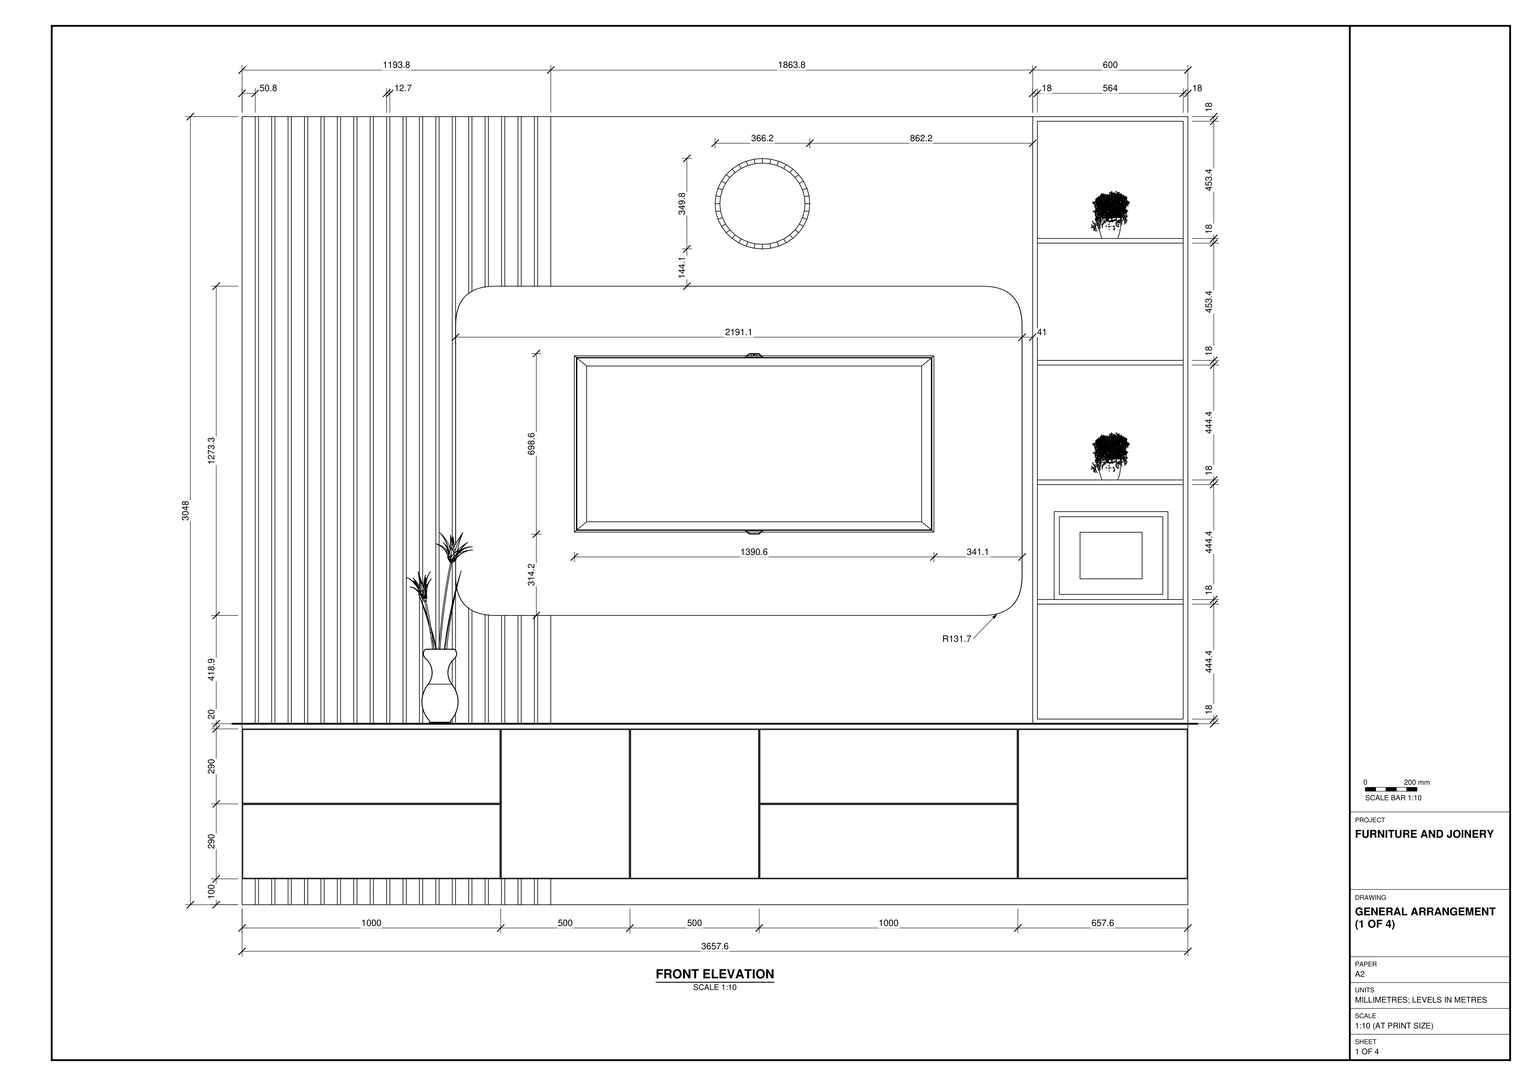
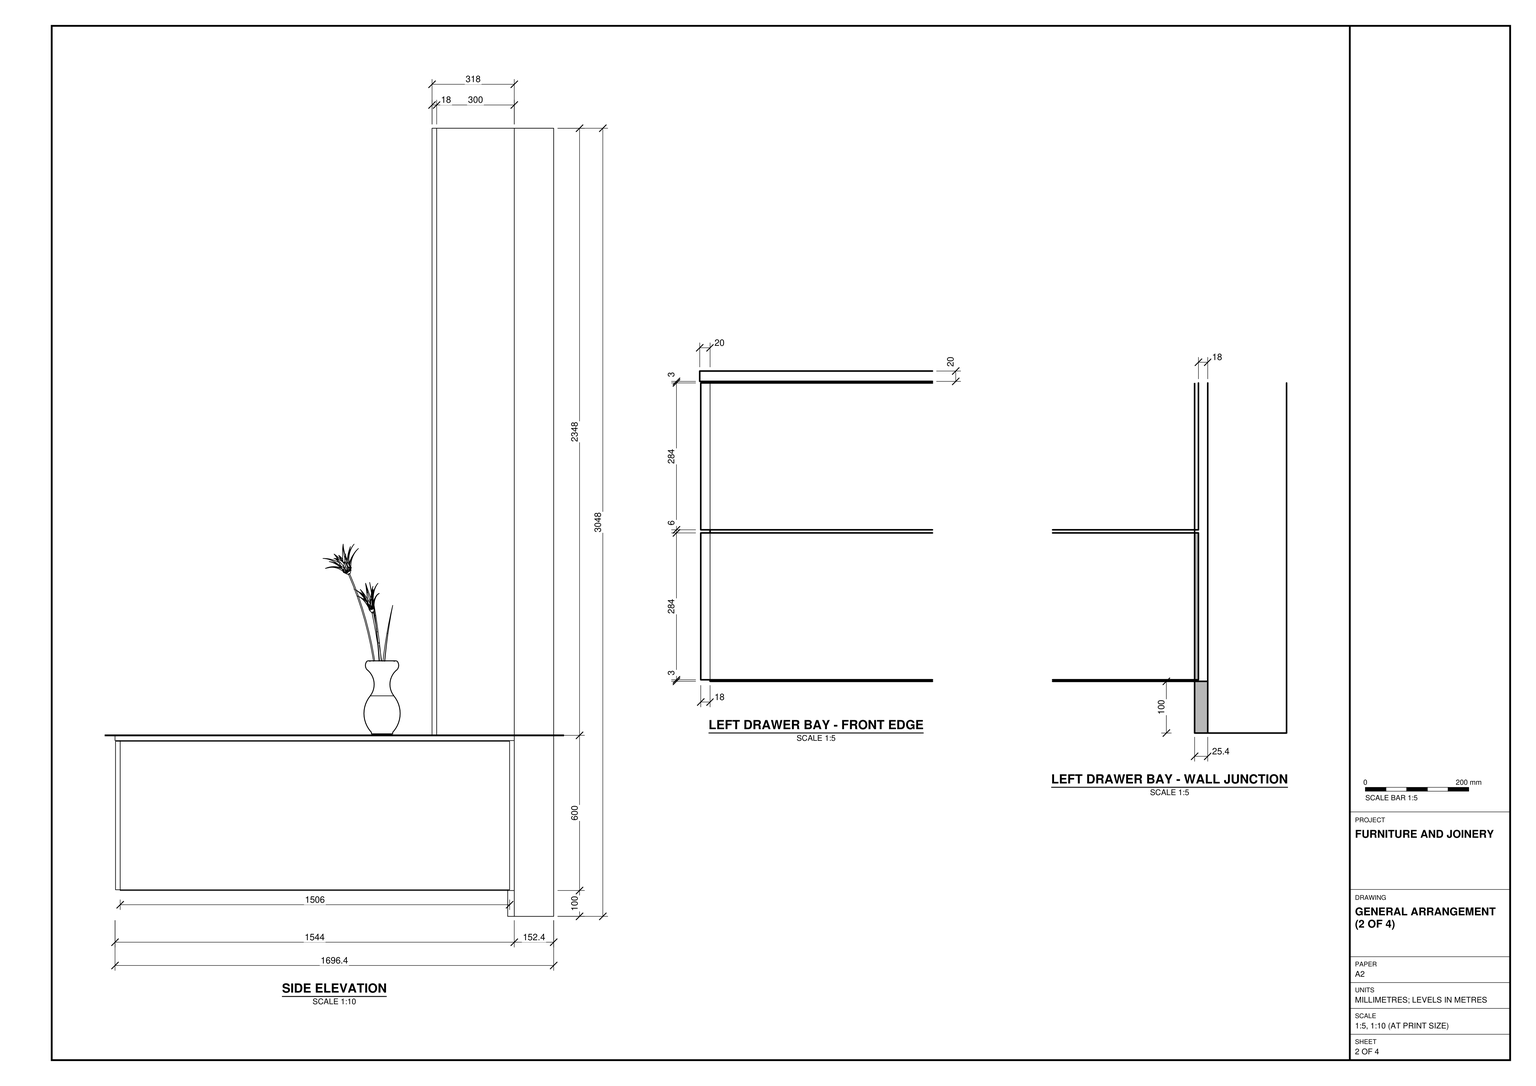
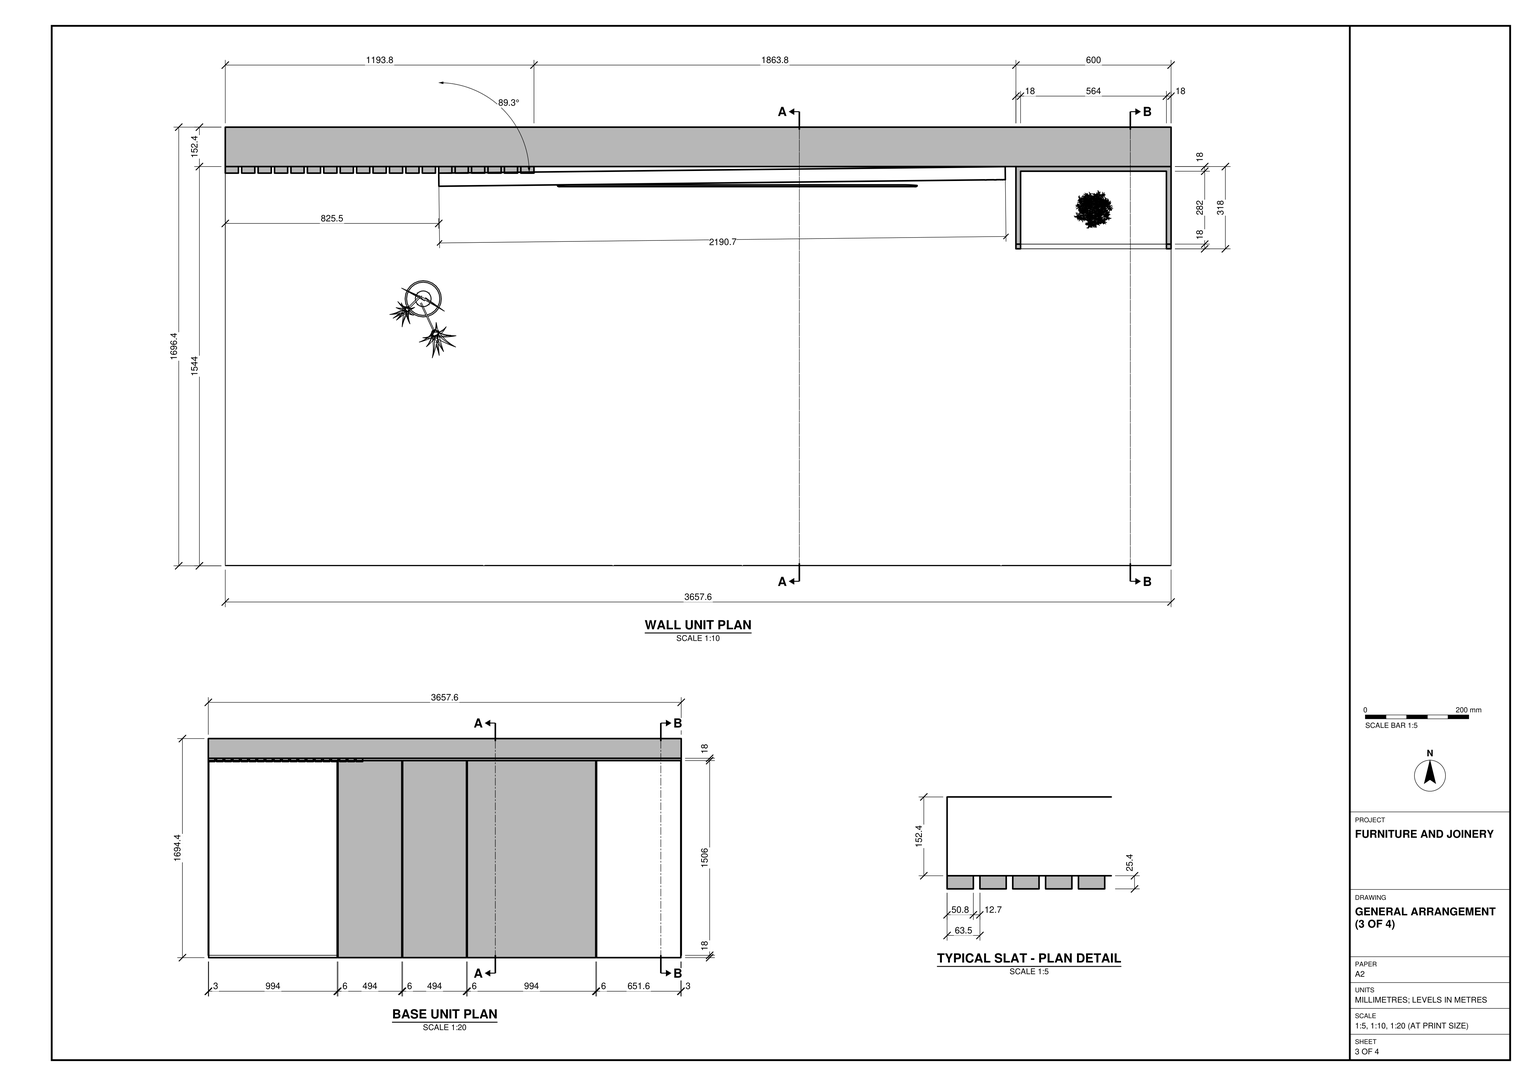
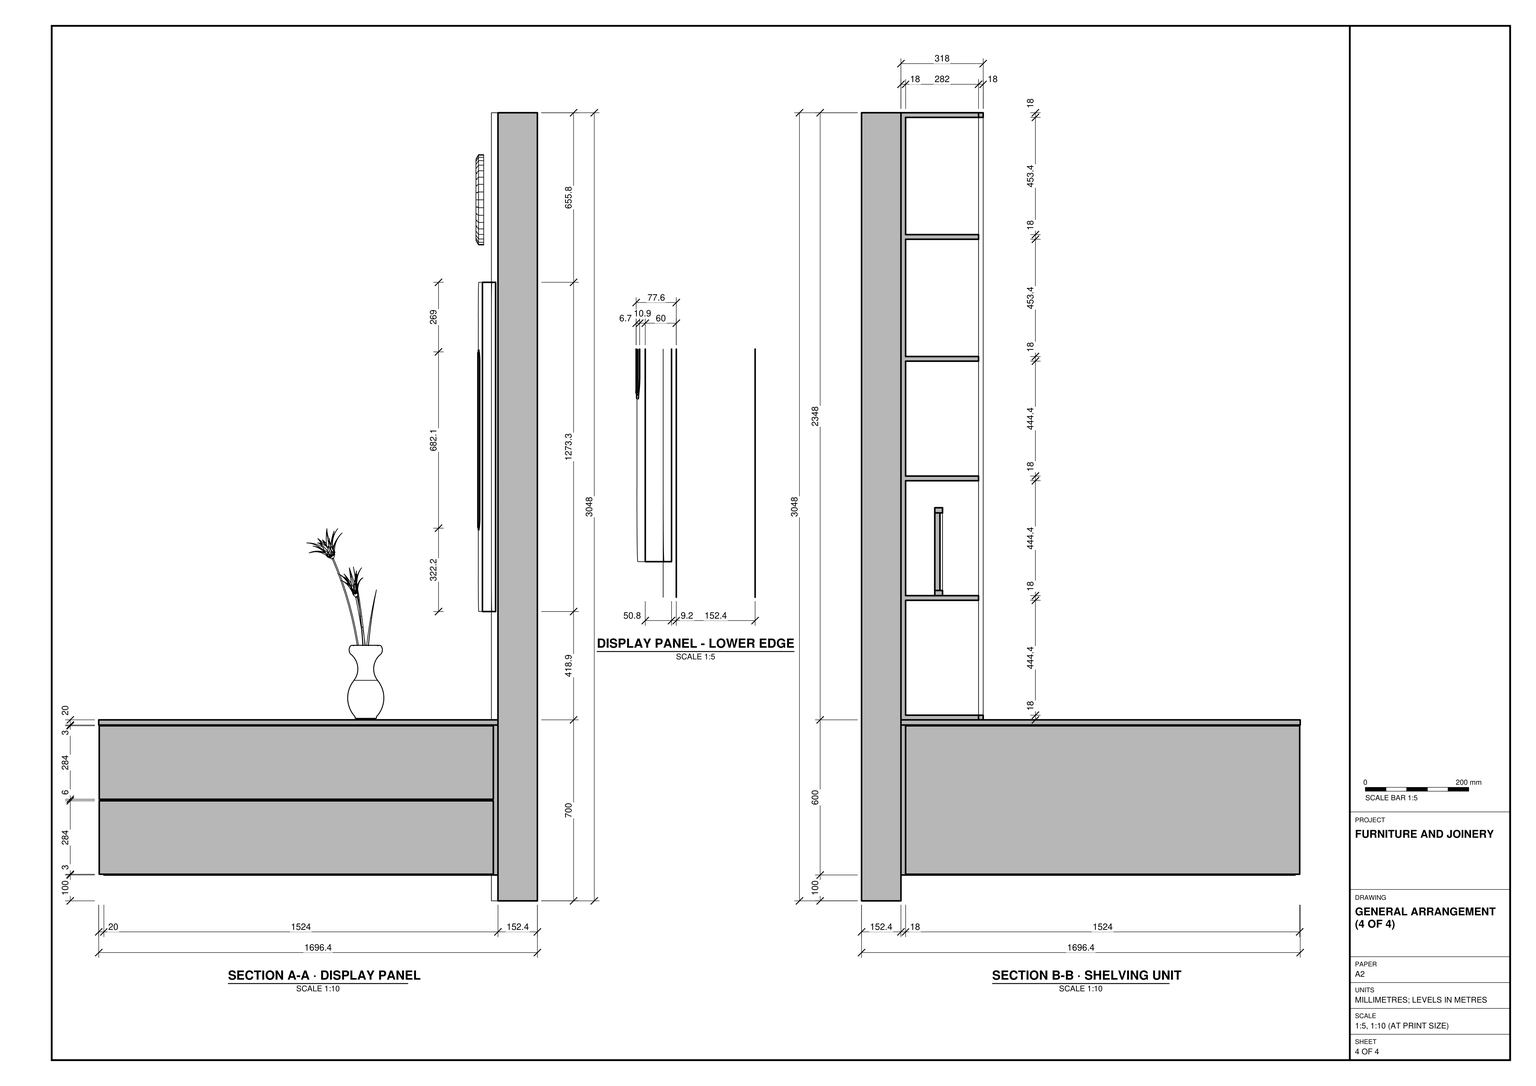
Build the TV wall unit in SketchUp from task_files/diagram_01.pdf. Work in millimetres, using the single floor level at 0 mm as the height datum. The complete assembly is 3657.6 mm wide, 1696.4 mm deep and 3048 mm high. Include the 152.4 mm thick backing wall; the overall depth includes this wall.

Run the base cabinetry across the full width, leaving its underside 100 mm above the floor. Model the continuous 20 mm thick top and follow the front elevation for the bay widths. The two wide bays have stacked drawer fronts, while the narrower bays have full-height fronts. Use the enlarged drawer detail for the gaps around the fronts.

On the left, model the vertical slats with the width, projection and clear spacing shown in the plan detail. Keep them visible below the base as well as above the top. Mount the rounded rectangular TV backing panel so that it overlaps the slatted field. Use the plan to set its slight angle to the wall. Place the TV on the panel, with the clock above it and the vase on the cabinet top to the left. At the right end, build the open shelving tower from the cabinet top to the top of the wall, following the shelf thicknesses and clear heights in the elevation. Place the plants and framed object in the indicated shelf openings. Decor and loose items may be any suitable library components.

Keep the backing wall and each distinct joinery or furniture piece in separate groups or components, and use components for repeated parts such as the slats. Save one SketchUp model as output_files/tv_wall_unit_with_base_cabinets_and_display_shelves.skp.

# SketchUp Ruby script. Lengths in millimetres.
U = 1.mm
M = Sketchup.active_model
def pt(a) = Geom::Point3d.new(a.map { |v| v * U })
def face(e, loops, mat)
  f = e.add_face(loops[0].map { |a| pt(a) })
  loops[1..].each { |l| e.add_face(l.map { |a| pt(a) }).erase! }
  f.material = f.back_material = mat if mat
  f
end
# faces: each face lists its corners as indices into pts; further lists are holes
def faces(e, pts, list, mat = nil) = list.each { |f| face(e, (f[0].is_a?(Array) ? f : [f]).map { |l| l.map { |i| pts[i] } }, mat) }
# xy, xz, yz: faces in a plane at the given z, y or x. An outline is a flat list of corners, or four numbers for a rectangle; further outlines are holes
def ring(l) = l.size == 4 ? [[l[0], l[1]], [l[2], l[1]], [l[2], l[3]], [l[0], l[3]]] : l.each_slice(2).to_a
def flat(e, list, mat, &to3) = list.each { |f| face(e, (f[0].is_a?(Array) ? f : [f]).map { |l| ring(l).map { |u, v| to3.(u, v) } }, mat) }
def xy(e, z, list, mat = nil) = flat(e, list, mat) { |x, y| [x, y, z] }
def xz(e, y, list, mat = nil) = flat(e, list, mat) { |x, z| [x, y, z] }
def yz(e, x, list, mat = nil) = flat(e, list, mat) { |y, z| [x, y, z] }
def lines(e, pts, list) = list.each { |a, b| e.add_line(pt(pts[a]), pt(pts[b])) }
# prism: a flat outline (further loops are holes) pulled along v
def prism(e, loops, v, mat = nil)
  f = face(e, loops, mat); d = Geom::Vector3d.new(v.map { |x| x * U })
  f.pushpull(f.normal.samedirection?(d) ? d.length : -d.length)
end
def box(e, o, s, mat = nil) = prism(e, [[o, [o[0] + s[0], o[1], o[2]], [o[0] + s[0], o[1] + s[1], o[2]], [o[0], o[1] + s[1], o[2]]]], [0, 0, s[2]], mat)
def at(x, y, z, deg = 0) = Geom::Transformation.translation(pt([x, y, z])) * Geom::Transformation.rotation(ORIGIN, Z_AXIS, deg.degrees)
def axes(o, x, y, z) = Geom::Transformation.new([*x, 0, *y, 0, *z, 0, *pt(o).to_a, 1])
def part(name) = M.definitions.add(name)
# library, detail: a bought-in or finely detailed component or shape, given as its bounding box
def library(name, o, s) = part(name).tap { |d| box(d.entities, o, s) }
def detail(e, o, s) = box(e.add_group.entities, o, s)
def put(e, d, t, mat = nil) = e.add_instance(d, t).tap { |i| i.material = mat if mat }
def group(e, t, mat = nil) = e.add_group.tap { |g| g.transformation = t; g.material = mat if mat }.entities
root = M.entities
M.materials.add("0297 AP 7187 LAVENDER SPRIG").color = [217, 213, 217]
M.materials.add("0301 AP 7183 GARDEN BEAUTY").color = [140, 140, 156]
M.materials.add("0303 AP 7181 VICTORIAN PURPLE").color = [80, 77, 85]
M.materials.add("[Carrera Marble]").color = [207, 207, 207]
M.materials.add("[Color_008]").color = [30, 30, 30]
M.materials.add("[Groundcover_RiverRock_4inch]").color = [145, 126, 109]
M.materials.add("[Wood Veneer 01]").color = [120, 70, 37]
c1 = part("Vertical wall slat")
xy(c1.entities,-3048,[[0,-25.4,50.8,0]],"0303 AP 7181 VICTORIAN PURPLE")
xy(c1.entities,0,[[0,-25.4,50.8,0]],"0303 AP 7181 VICTORIAN PURPLE")
xz(c1.entities,-25.4,[[0,-3048,50.8,0]],"0303 AP 7181 VICTORIAN PURPLE")
xz(c1.entities,0,[[0,-3048,50.8,0]],"[Wood Veneer 01]")
yz(c1.entities,0,[[-25.4,-3048,0,0]],"0303 AP 7181 VICTORIAN PURPLE")
yz(c1.entities,50.8,[[-25.4,-3048,0,0]],"0303 AP 7181 VICTORIAN PURPLE")
c2 = library("Flat screen television",[0,35.9,29],[912.5,6.9,513.2])
c3 = library("Hodiny",[0,0,0],[300,30,300])
c4 = library("Potted plant",[-6.2,-40.8,0],[184.7,184.7,183.2])
c5 = part("Framed picture")
xy(c5.entities,0,[[[-20,-20,420,320],[0,0,400,300]],[[0,0,400,300],[80,60,320,240]]])
xy(c5.entities,20,[[[0,0,400,300],[80,60,320,240]]])
xy(c5.entities,30,[[[-20,-20,420,320],[0,0,400,300]]],"[Color_008]")
xz(c5.entities,-20,[[-20,0,420,30]],"[Color_008]")
xz(c5.entities,0,[[0,0,400,20]])
xz(c5.entities,0,[[0,20,400,30]],"[Color_008]")
xz(c5.entities,60,[[80,0,320,20]])
xz(c5.entities,240,[[80,0,320,20]])
xz(c5.entities,300,[[0,0,400,20]])
xz(c5.entities,300,[[0,20,400,30]],"[Color_008]")
xz(c5.entities,320,[[-20,0,420,30]],"[Color_008]")
yz(c5.entities,-20,[[-20,0,320,30]],"[Color_008]")
yz(c5.entities,0,[[0,0,300,20]])
yz(c5.entities,0,[[0,20,300,30]],"[Color_008]")
yz(c5.entities,80,[[60,0,240,20]])
yz(c5.entities,320,[[60,0,240,20]])
yz(c5.entities,400,[[0,0,300,20]])
yz(c5.entities,400,[[0,20,300,30]],"[Color_008]")
yz(c5.entities,420,[[-20,0,320,30]],"[Color_008]")
g1 = group(c5.entities,at(0,0,20))
xy(g1,0,[[80,60,320,240]],"[Groundcover_RiverRock_4inch]")
c6 = library("Group\#20",[-267.8,-620.3,-14],[1019,1090.2,2508.2])
put(root,c1,at(0,1544,3048))
put(root,c1,at(63.5,1544,3048))
put(root,c1,at(127,1544,3048))
put(root,c1,at(190.5,1544,3048))
put(root,c1,at(254,1544,3048))
put(root,c1,at(317.5,1544,3048))
put(root,c1,at(381,1544,3048))
put(root,c1,at(444.5,1544,3048))
put(root,c1,at(508,1544,3048))
put(root,c1,at(571.5,1544,3048))
put(root,c1,at(635,1544,3048))
put(root,c1,at(698.5,1544,3048))
put(root,c1,at(762,1544,3048))
put(root,c1,at(825.5,1544,3048))
put(root,c1,at(889,1544,3048))
put(root,c1,at(952.5,1544,3048))
put(root,c1,at(1016,1544,3048))
put(root,c1,at(1079.5,1544,3048))
put(root,c1,at(1143,1544,3048))
put(root,c2,axes([1284.8,1430.3,1393.6],[1.524,0,0],[0,1,0],[0,0,1.36127]))
put(root,c3,axes([1829.2,1458.8,2536.3],[1.2208,0,0],[0,1,0],[0,0,1.166]))
put(root,c4,at(3273.8,1324.2,2576.6))
put(root,c4,at(3273.8,1324.2,1642.8))
put(root,c5,axes([3160.6,1413.1,1200.4],[1,0,0],[0,0,1],[0,-1,0]))
g2 = group(root,at(0,1544,0),"0297 AP 7187 LAVENDER SPRIG")
xy(g2,0,[[0,0,3657.6,152.4]])
xy(g2,3048,[[0,0,3657.6,152.4]])
xz(g2,0,[[0,0,3657.6,3048]],"0297 AP 7187 LAVENDER SPRIG")
xz(g2,152.4,[[0,0,3657.6,3048]],"0297 AP 7187 LAVENDER SPRIG")
yz(g2,0,[[0,0,152.4,3048]])
yz(g2,3657.6,[[0,0,152.4,3048]],"0297 AP 7187 LAVENDER SPRIG")
g3 = group(root,at(0,0,100))
g4 = group(g3,at(0,2,0),"0301 AP 7183 GARDEN BEAUTY")
xy(g4,3,[[3,0,997,18]])
xy(g4,287,[[3,0,997,18]])
xz(g4,0,[[3,3,997,287]])
xz(g4,18,[[[0,0,1000,290],[3,3,997,287]]])
yz(g4,3,[[0,3,18,287]])
yz(g4,997,[[0,3,18,287]])
g5 = group(g3,at(0,20,0),"[Carrera Marble]")
xy(g5,0,[[0,0,3657.6,1524]])
xy(g5,3,[[3,0,997,1506],[1003,0,1497,1506],[1503,0,1997,1506],[2003,0,2997,1506],[3003,0,3654.6,1506]])
xy(g5,287,[[3,0,997,1506],[2003,0,2997,1506]])
xy(g5,293,[[3,0,997,1506],[2003,0,2997,1506]])
xy(g5,577,[[3,0,997,1506],[1003,0,1497,1506],[1503,0,1997,1506],[2003,0,2997,1506],[3003,0,3654.6,1506]])
xy(g5,580,[[0,-20,3657.6,0],[0,0,3657.6,1524]])
xy(g5,600,[[0,-20,3657.6,1524]])
xz(g5,-20,[[0,580,3657.6,600]])
xz(g5,0,[[[0,0,1000,290],[3,3,997,287]],[[1000,0,1500,580],[1003,3,1497,577]],[[1500,0,2000,580],[1503,3,1997,577]],[[2000,0,3000,290],[2003,3,2997,287]],[[3000,0,3657.6,580],[3003,3,3654.6,577]],
  [[0,290,1000,580],[3,293,997,577]],[[2000,290,3000,580],[2003,293,2997,577]]])
xz(g5,1506,[[3,3,997,287],[1003,3,1497,577],[1503,3,1997,577],[2003,3,2997,287],[3003,3,3654.6,577],
  [3,293,997,577],[2003,293,2997,577]])
xz(g5,1524,[[0,0,3657.6,580],[0,580,3657.6,600]])
yz(g5,0,[[0,0,1524,580],[-20,580,1524,600]])
yz(g5,3,[[0,3,1506,287],[0,293,1506,577]])
yz(g5,997,[[0,3,1506,287],[0,293,1506,577]])
yz(g5,1003,[[0,3,1506,290],[0,290,1506,577]])
yz(g5,1497,[[0,3,1506,577]])
yz(g5,1503,[[0,3,1506,577]])
yz(g5,1997,[[0,3,1506,577]])
yz(g5,2003,[[0,3,1506,287],[0,293,1506,577]])
yz(g5,2997,[[0,3,1506,287],[0,293,1506,577]])
yz(g5,3003,[[0,3,1506,290],[0,290,1506,577]])
yz(g5,3654.6,[[0,3,1506,577]])
yz(g5,3657.6,[[0,0,1524,580],[-20,580,1524,600]])
g6 = group(g3,at(0,2,290),"0301 AP 7183 GARDEN BEAUTY")
xy(g6,3,[[3,0,997,18]])
xy(g6,287,[[3,0,997,18]])
xz(g6,0,[[3,3,997,287]])
xz(g6,18,[[[0,0,1000,290],[3,3,997,287]]])
yz(g6,3,[[0,3,18,287]])
yz(g6,997,[[0,3,18,287]])
g7 = group(g3,at(1000,2,0),"0301 AP 7183 GARDEN BEAUTY")
xy(g7,3,[[3,0,497,18]])
xy(g7,577,[[3,0,497,18]])
xz(g7,0,[[3,3,497,577]])
xz(g7,18,[[[0,0,500,580],[3,3,497,577]]])
yz(g7,3,[[0,3,18,577]])
yz(g7,497,[[0,3,18,577]])
g8 = group(g3,at(1999.8,2,290),"0301 AP 7183 GARDEN BEAUTY")
xy(g8,3,[[3,0,997.2,18]])
xy(g8,287.2,[[3,0,997.2,18]])
xz(g8,0,[[3,3,997.2,287.2]])
xz(g8,18,[[[0,0,1000.2,290.2],[3,3,997.2,287.2]]])
yz(g8,3,[[0,3,18,287.2]])
yz(g8,997.2,[[0,3,18,287.2]])
g9 = group(g3,at(2000,2,0),"0301 AP 7183 GARDEN BEAUTY")
xy(g9,3,[[3,0,997,18]])
xy(g9,287,[[3,0,997,18]])
xz(g9,0,[[3,3,997,287]])
xz(g9,18,[[[0,0,1000,290],[3,3,997,287]]])
yz(g9,3,[[0,3,18,287]])
yz(g9,997,[[0,3,18,287]])
g10 = group(g3,at(3000,2,0),"0301 AP 7183 GARDEN BEAUTY")
xy(g10,3,[[3,0,654.6,18]])
xy(g10,577,[[3,0,654.6,18]])
xz(g10,0,[[3,3,654.6,577]])
xz(g10,18,[[[0,0,657.6,580],[3,3,654.6,577]]])
yz(g10,3,[[0,3,18,577]])
yz(g10,654.6,[[0,3,18,577]])
g11 = group(g3,at(1500,2,0),"0301 AP 7183 GARDEN BEAUTY")
xy(g11,3,[[3,0,497,18]])
xy(g11,577,[[3,0,497,18]])
xz(g11,0,[[3,3,497,577]])
xz(g11,18,[[[0,0,500,580],[3,3,497,577]]])
yz(g11,3,[[0,3,18,577]])
yz(g11,497,[[0,3,18,577]])
g12 = group(root,at(3057.6,1244,700),"0303 AP 7181 VICTORIAN PURPLE")
xy(g12,0,[[0,-18,600,0],[0,0,600,300]])
xy(g12,18,[[18,-18,582,0],[18,0,582,282]])
xy(g12,462.4,[[18,0,582,282]])
xy(g12,480.4,[[18,0,582,282]])
xy(g12,924.8,[[18,0,582,282]])
xy(g12,942.8,[[18,0,582,282]])
xy(g12,1387.2,[[18,0,582,282]])
xy(g12,1405.2,[[18,0,582,282]])
xy(g12,1858.6,[[18,0,582,282]])
xy(g12,1876.6,[[18,0,582,282]])
xy(g12,2330,[[18,-18,582,0],[18,0,582,282]])
xy(g12,2348,[[0,-18,600,0],[0,0,600,300]])
xz(g12,-18,[[[0,0,600,2348],[18,18,582,2330]]])
xz(g12,0,[[[0,0,600,2348],[18,18,582,2330]],[18,462.4,582,480.4],[18,924.8,582,942.8],[18,1387.2,582,1405.2],[18,1858.6,582,1876.6]])
xz(g12,282,[[18,18,582,462.4],[18,480.4,582,924.8],[18,942.8,582,1387.2],[18,1405.2,582,1858.6],[18,1876.6,582,2330]])
xz(g12,300,[[0,0,600,2348]])
yz(g12,0,[[-18,0,0,2348],[0,0,300,2348]])
yz(g12,18,[[-18,18,0,2330],[0,18,282,462.4],[0,480.4,282,924.8],[0,942.8,282,1387.2],[0,1405.2,282,1858.6],
  [0,1876.6,282,2330]])
yz(g12,582,[[-18,18,0,2330],[0,18,282,462.4],[0,480.4,282,924.8],[0,942.8,282,1387.2],[0,1405.2,282,1858.6],
  [0,1876.6,282,2330]])
yz(g12,600,[[-18,0,0,2348],[0,0,300,2348]])
g13 = group(root,at(825.5,1467.8,1118.9))
prism(g13,[[[0,50.8,1120.9],[0.3,50.8,1133.3],[1.1,50.8,1145.2],[2.4,50.8,1156.6],[4.2,50.8,1167.4],[6.6,50.9,1177.8],[9.5,50.9,1187.5],[13,50.9,1196.8],[16.9,51,1205.5],[21.4,51,1213.7],[26.5,51.1,1221.4],[32,51.2,1228.6],[38.1,51.2,1235.2],[44.7,51.3,1241.3],[51.9,51.4,1246.8],[59.5,51.5,1251.8],[67.7,51.6,1256.3],[76.5,51.7,1260.3],[85.7,51.8,1263.7],[95.5,51.9,1266.7],[105.8,52,1269],[116.7,52.1,1270.9],[128,52.3,1272.2],[140,52.4,1273],[152.4,52.6,1273.3],[2038.1,74.4,1273.3],[2050.6,74.6,1273],[2062.5,74.7,1272.2],[2073.8,74.8,1270.9],[2084.7,75,1269],[2095,75.1,1266.7],[2104.8,75.2,1263.7],[2114,75.3,1260.3],[2122.8,75.4,1256.3],[2131,75.5,1251.8],[2138.7,75.6,1246.8],[2145.8,75.7,1241.3],[2152.4,75.8,1235.2],[2158.5,75.8,1228.6],[2164,75.9,1221.4],[2169.1,75.9,1213.7],[2173.6,76,1205.5],[2177.5,76,1196.8],[2181,76.1,1187.5],[2183.9,76.1,1177.8],[2186.3,76.1,1167.4],[2188.1,76.2,1156.6],[2189.4,76.2,1145.2],[2190.2,76.2,1133.3],[2190.5,76.2,1120.9],[2190.5,76.2,152.4],[2190.2,76.2,140],[2189.4,76.2,128.1],[2188.1,76.2,116.7],[2186.3,76.1,105.8],[2183.9,76.1,95.5],[2181,76.1,85.7],[2177.5,76,76.5],[2173.6,76,67.7],[2169.1,75.9,59.5],[2164,75.9,51.9],[2158.5,75.8,44.7],[2152.4,75.8,38.1],[2145.8,75.7,32],[2138.7,75.6,26.5],[2131,75.5,21.4],[2122.8,75.4,16.9],[2114,75.3,13],[2104.8,75.2,9.5],[2095,75.1,6.6],[2084.7,75,4.2],[2073.8,74.8,2.4],[2062.5,74.7,1.1],[2050.6,74.6,0.3],[2038.1,74.4,0],[152.4,52.6,0],[140,52.4,0.3],[128,52.3,1.1],[116.7,52.1,2.4],[105.8,52,4.2],[95.5,51.9,6.6],[85.7,51.8,9.5],[76.5,51.7,13],[67.7,51.6,16.9],[59.5,51.5,21.4],[51.9,51.4,26.5],[44.7,51.3,32],[38.1,51.2,38.1],[32,51.2,44.7],[26.5,51.1,51.9],[21.4,51,59.5],[16.9,51,67.7],[13,50.9,76.5],[9.5,50.9,85.7],[6.6,50.9,95.5],[4.2,50.8,105.8],[2.4,50.8,116.7],[1.1,50.8,128.1],[0.3,50.8,140],[0,50.8,152.4]]],[0.6,-50.8,0])
put(root,c6,axes([695,962.2,704.2],[0.3,0,0],[0,0.3,0],[0,0,0.3]))
